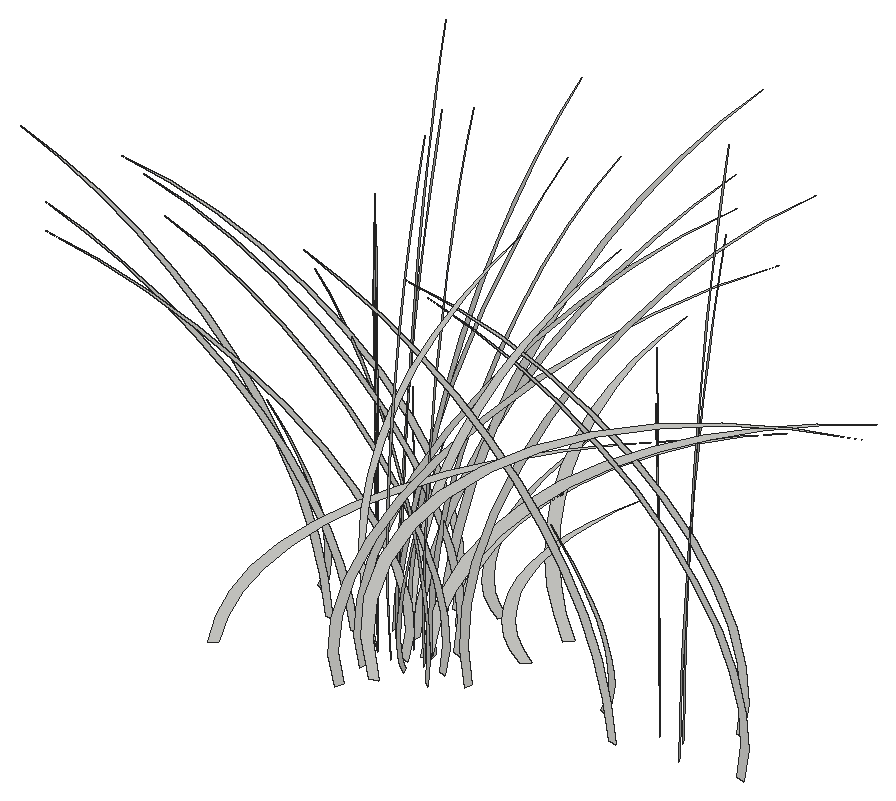
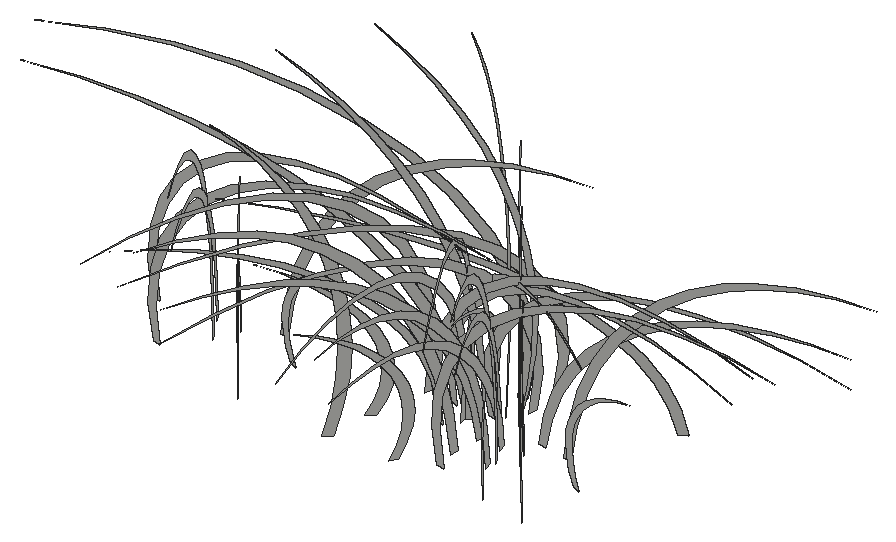
# SketchUp Ruby script. Lengths in inches.
U = 1.inch
M = Sketchup.active_model
def pt(a) = Geom::Point3d.new(a.map { |v| v * U })
def face(e, loops, mat)
  f = e.add_face(loops[0].map { |a| pt(a) })
  loops[1..].each { |l| e.add_face(l.map { |a| pt(a) }).erase! }
  f.material = f.back_material = mat if mat
  f
end
# faces: each face lists its corners as indices into pts; further lists are holes
def faces(e, pts, list, mat = nil) = list.each { |f| face(e, (f[0].is_a?(Array) ? f : [f]).map { |l| l.map { |i| pts[i] } }, mat) }
# xy, xz, yz: faces in a plane at the given z, y or x. An outline is a flat list of corners, or four numbers for a rectangle; further outlines are holes
def ring(l) = l.size == 4 ? [[l[0], l[1]], [l[2], l[1]], [l[2], l[3]], [l[0], l[3]]] : l.each_slice(2).to_a
def flat(e, list, mat, &to3) = list.each { |f| face(e, (f[0].is_a?(Array) ? f : [f]).map { |l| ring(l).map { |u, v| to3.(u, v) } }, mat) }
def xy(e, z, list, mat = nil) = flat(e, list, mat) { |x, y| [x, y, z] }
def xz(e, y, list, mat = nil) = flat(e, list, mat) { |x, z| [x, y, z] }
def yz(e, x, list, mat = nil) = flat(e, list, mat) { |y, z| [x, y, z] }
def lines(e, pts, list) = list.each { |a, b| e.add_line(pt(pts[a]), pt(pts[b])) }
# prism: a flat outline (further loops are holes) pulled along v
def prism(e, loops, v, mat = nil)
  f = face(e, loops, mat); d = Geom::Vector3d.new(v.map { |x| x * U })
  f.pushpull(f.normal.samedirection?(d) ? d.length : -d.length)
end
def box(e, o, s, mat = nil) = prism(e, [[o, [o[0] + s[0], o[1], o[2]], [o[0] + s[0], o[1] + s[1], o[2]], [o[0], o[1] + s[1], o[2]]]], [0, 0, s[2]], mat)
def at(x, y, z, deg = 0) = Geom::Transformation.translation(pt([x, y, z])) * Geom::Transformation.rotation(ORIGIN, Z_AXIS, deg.degrees)
def axes(o, x, y, z) = Geom::Transformation.new([*x, 0, *y, 0, *z, 0, *pt(o).to_a, 1])
def part(name) = M.definitions.add(name)
# library, detail: a bought-in or finely detailed component or shape, given as its bounding box
def library(name, o, s) = part(name).tap { |d| box(d.entities, o, s) }
def detail(e, o, s) = box(e.add_group.entities, o, s)
def put(e, d, t, mat = nil) = e.add_instance(d, t).tap { |i| i.material = mat if mat }
def group(e, t, mat = nil) = e.add_group.tap { |g| g.transformation = t; g.material = mat if mat }.entities
root = M.entities
g1 = group(root,at(381.84,271.38,0))
p = [[-20.46,3.64,18.05],[-23.54,4.19,18.53],[-20.55,3.66,17.95],[-17.67,3.15,17.15],[-14.91,2.66,16.14],[-12.33,2.2,14.93],
  [-9.93,1.77,13.53],[-7.76,1.38,11.96],[-5.84,1.04,10.23],[-4.18,0.74,8.37],[-2.8,0.5,6.39],[-1.73,0.31,4.32],
  [-0.97,0.17,2.18],[-0.53,0.09,0],[0,0,0],[-0.36,0.0625,2.23],[-1.07,0.19,4.43],[-2.125,0.38,6.55],
  [-3.51,0.625,8.57],[-5.2,0.93,10.47],[-7.1875,1.28,12.22],[-9.43,1.68,13.8],[-11.92,2.125,15.1875],[-14.61,2.6,16.37],
  [-17.46,3.11,17.33]]
faces(g1,p,[[0,1,2,3,4,5,6,7,8,9,10,11,12,13,14,15,16,17,18,19,20,21,22,23,24]])
g2 = group(root,at(359.18,266.76,0.02))
p = [[17.17,11.7,12.375],[19.76,13.47,12.7],[17.25,11.76,12.31],[14.83,10.11,11.76],[12.52,8.53,11.07],[10.35,7.05,10.23],
  [8.34,5.68,9.27],[6.52,4.44,8.2],[4.9,3.34,7.01],[3.51,2.39,5.74],[2.35,1.6,4.38],[1.45,0.99,2.96],
  [0.82,0.56,1.5],[0.45,0.3,0],[0,0,0],[0.3,0.21,1.53],[0.9,0.61,3.03],[1.78,1.22,4.49],
  [2.95,2.01,5.875],[4.37,2.98,7.18],[6.03,4.11,8.375],[7.92,5.4,9.46],[10,6.82,10.41],[12.26,8.36,11.22],
  [14.66,9.99,11.88]]
faces(g2,p,[[0,1,2,3,4,5,6,7,8,9,10,11,12,13,14,15,16,17,18,19,20,21,22,23,24]])
g3 = group(root,at(365.85,270.62,0.02))
p = [[0.67,0.67,0],[0.3,0.3,2.04],[0.08,0.08,4.1],[0,0,6.17],[0.07,0.07,8.23],[0.3,0.3,10.29],
  [0.66,0.66,12.33],[1.18,1.18,14.34],[1.84,1.84,16.32],[2.64,2.64,18.26],[3.58,3.58,20.14],[4.65,4.65,21.96],
  [5.84,5.84,23.71],[4.72,4.72,21.93],[3.71,3.71,20.09],[2.82,2.82,18.2],[2.05,2.05,16.26],[1.42,1.42,14.29],
  [0.91,0.91,12.29],[0.54,0.54,10.26],[0.3,0.3,8.21],[0.1875,0.1875,6.15],[0.22,0.22,4.09],[0.375,0.375,2.04]]
faces(g3,p,[[0,1,2,3,4,5,6,7,8,9,10,11,12,13,14,15,16,17,18,19,20,21,22,23]])
g4 = group(root,at(369.38,269.29,0.02))
p = [[-3.85,8.68,9.0625],[-3.11,7.03,8.49],[-2.45,5.54,7.85],[-1.87,4.22,7.18],[-1.37,3.08,6.45],[-0.95,2.15,5.7],
  [-0.625,1.41,4.91],[-0.39,0.89,4.1],[-0.26,0.58,3.28],[-0.22,0.49,2.45],[-0.28,0.625,1.625],[-0.43,0.97,0.8],
  [-0.68,1.54,0],[-0.52,1.16,0],[-0.23,0.52,0.8],[-0.05,0.11,1.61],[0.02,-0.06,2.45],[-0.01,0.02,3.28],
  [-0.15,0.33,4.11],[-0.39,0.89,4.93],[-0.74,1.67,5.72],[-1.1875,2.68,6.49],[-1.73,3.9,7.21],[-2.35,5.3125,7.88],
  [-3.0625,6.91,8.5]]
faces(g4,p,[[0,1,2,3,4,5,6,7,8,9,10,11,12,13,14,15,16,17,18,19,20,21,22,23,24]])
g5 = group(root,at(367.54,268.67,0.02))
p = [[0.85,0.36,0],[0.38,0.16,0],[0,0,2.37],[0.15,0.0625,4.75],[0.84,0.35,7.08],[2.03,0.85,9.32],
  [3.71,1.54,11.39],[5.83,2.42,13.25],[8.33,3.47,14.85],[11.16,4.65,16.15],[14.25,5.93,17.13],[17.52,7.29,17.75],
  [20.89,8.69,18.01],[24.27,10.1,17.89],[20.95,8.72,17.91],[17.67,7.35,17.58],[14.49,6.03,16.9],[11.5,4.79,15.89],
  [8.76,3.65,14.58],[6.33,2.63,12.99],[4.27,1.78,11.15],[2.63,1.1,9.125],[1.45,0.6,6.94],[0.75,0.3125,4.66],
  [0.55,0.23,2.33]]
faces(g5,p,[[0,1,2,3,4,5,6,7,8,9,10,11,12,13,14,15,16,17,18,19,20,21,22,23,24]])
g6 = group(root,at(367.12,270.56,0.02))
p = [[-0.6,0.73,0],[-0.27,0.33,1.77],[-0.07,0.08,3.57],[0,0,5.36],[-0.07,0.08,7.16],[-0.27,0.32,8.95],
  [-0.6,0.73,10.73],[-1.06,1.29,12.48],[-1.65,2.01,14.2],[-2.37,2.88,15.88],[-3.21,3.91,17.52],[-4.17,5.08,19.1],
  [-5.25,6.39,20.625],[-4.23,5.15,19.08],[-3.33,4.05,17.48],[-2.53,3.08,15.83],[-1.84,2.25,14.15],[-1.27,1.55,12.43],
  [-0.82,1,10.6875],[-0.48,0.59,8.92],[-0.27,0.32,7.14],[-0.17,0.21,5.35],[-0.19,0.24,3.5625],[-0.34,0.41,1.78]]
faces(g6,p,[[0,1,2,3,4,5,6,7,8,9,10,11,12,13,14,15,16,17,18,19,20,21,22,23]])
g7 = group(root,at(368.81,271.35,0.02))
p = [[-0.98,0.17,0],[-0.43,0.08,0],[0,0,1.75],[-0.18,0.03,3.51],[-0.96,0.17,5.24],[-2.32,0.41,6.89],
  [-4.24,0.76,8.42],[-6.67,1.1875,9.8],[-9.54,1.7,10.98],[-12.78,2.28,11.95],[-16.32,2.91,12.67],[-20.06,3.57,13.13],
  [-23.91,4.26,13.32],[-27.78,4.95,13.23],[-23.98,4.27,13.25],[-20.22,3.6,13],[-16.59,2.96,12.5],[-13.16,2.34,11.75],
  [-10.02,1.79,10.78],[-7.25,1.29,9.6],[-4.89,0.87,8.25],[-3.02,0.54,6.75],[-1.66,0.3,5.13],[-0.86,0.15,3.44],
  [-0.63,0.11,1.72]]
faces(g7,p,[[0,1,2,3,4,5,6,7,8,9,10,11,12,13,14,15,16,17,18,19,20,21,22,23,24]])
g8 = group(root,at(368.81,271.35,0.02))
p = [[-0.98,0.17,0],[-0.43,0.08,0],[0,0,1.75],[-0.18,0.03,3.51],[-0.96,0.17,5.24],[-2.32,0.41,6.89],
  [-4.24,0.76,8.42],[-6.67,1.1875,9.8],[-9.54,1.7,10.98],[-12.78,2.28,11.95],[-16.32,2.91,12.67],[-20.06,3.57,13.13],
  [-23.91,4.26,13.32],[-27.78,4.95,13.23],[-23.98,4.27,13.25],[-20.22,3.6,13],[-16.59,2.96,12.5],[-13.16,2.34,11.75],
  [-10.02,1.79,10.78],[-7.25,1.29,9.6],[-4.89,0.87,8.25],[-3.02,0.54,6.75],[-1.66,0.3,5.13],[-0.86,0.15,3.44],
  [-0.63,0.11,1.72]]
faces(g8,p,[[0,1,2,3,4,5,6,7,8,9,10,11,12,13,14,15,16,17,18,19,20,21,22,23,24]])
g9 = group(root,at(367.92,270.26,0.02))
p = [[-0.4,0.86,0],[-0.18,0.38,2.26],[-0.05,0.1,4.55],[0,0,6.84],[-0.04,0.09,9.14],[-0.18,0.38,11.42],
  [-0.4,0.85,13.6875],[-0.71,1.51,15.92],[-1.1,2.36,18.12],[-1.58,3.38,20.26],[-2.14,4.58,22.35],[-2.79,5.95,24.37],
  [-3.51,7.48,26.3125],[-2.83,6.04,24.34],[-2.22,4.75,22.3],[-1.69,3.61,20.2],[-1.23,2.63,18.05],[-0.85,1.82,15.86],
  [-0.55,1.17,13.64],[-0.32,0.6875,11.38],[-0.18,0.38,9.11],[-0.11,0.24,6.83],[-0.13,0.28,4.54],[-0.23,0.48,2.27]]
faces(g9,p,[[0,1,2,3,4,5,6,7,8,9,10,11,12,13,14,15,16,17,18,19,20,21,22,23]])
g10 = group(root,at(364.57,272.11,0.02))
p = [[-20.46,3.64,14.56],[-23.54,4.19,14.94],[-20.55,3.66,14.48],[-17.67,3.15,13.83],[-14.91,2.66,13.02],[-12.33,2.2,12.04],
  [-9.93,1.77,10.91],[-7.76,1.38,9.64],[-5.84,1.04,8.25],[-4.18,0.74,6.75],[-2.8,0.5,5.15],[-1.73,0.31,3.49],
  [-0.97,0.17,1.76],[-0.53,0.09,0],[0,0,0],[-0.36,0.0625,1.8],[-1.07,0.19,3.57],[-2.125,0.38,5.28],
  [-3.51,0.625,6.91],[-5.2,0.93,8.44],[-7.1875,1.28,9.85],[-9.43,1.68,11.13],[-11.92,2.125,12.25],[-14.61,2.6,13.2],
  [-17.46,3.11,13.97]]
faces(g10,p,[[0,1,2,3,4,5,6,7,8,9,10,11,12,13,14,15,16,17,18,19,20,21,22,23,24]])
g11 = group(root,at(362.67,272.45,0.02))
p = [[-20.46,3.64,18.05],[-23.54,4.19,18.53],[-20.55,3.66,17.95],[-17.67,3.15,17.15],[-14.91,2.66,16.14],[-12.33,2.2,14.93],
  [-9.93,1.77,13.53],[-7.76,1.38,11.96],[-5.84,1.04,10.23],[-4.18,0.74,8.37],[-2.8,0.5,6.39],[-1.73,0.31,4.32],
  [-0.97,0.17,2.18],[-0.53,0.09,0],[0,0,0],[-0.36,0.0625,2.23],[-1.07,0.19,4.43],[-2.125,0.38,6.55],
  [-3.51,0.625,8.57],[-5.2,0.93,10.47],[-7.1875,1.28,12.22],[-9.43,1.68,13.8],[-11.92,2.125,15.1875],[-14.61,2.6,16.37],
  [-17.46,3.11,17.33]]
faces(g11,p,[[0,1,2,3,4,5,6,7,8,9,10,11,12,13,14,15,16,17,18,19,20,21,22,23,24]])
g12 = group(root,at(380.4,273.07,0))
p = [[-6.53,2.99,7.88],[-5.33,2.44,7.38],[-4.26,1.95,6.83],[-3.3,1.51,6.24],[-2.48,1.14,5.62],[-1.81,0.83,4.96],
  [-1.28,0.58,4.27],[-0.9,0.41,3.57],[-0.68,0.31,2.86],[-0.61,0.28,2.13],[-0.71,0.32,1.41],[-0.96,0.4375,0.7],
  [-1.37,0.625,0],[-0.84,0.38,0],[-0.39,0.18,0.71],[-0.11,0.05,1.43],[0,0,2.17],[-0.07,0.03,2.9],
  [-0.32,0.15,3.63],[-0.74,0.34,4.34],[-1.33,0.61,5.03],[-2.08,0.95,5.69],[-2.99,1.37,6.3125],[-4.04,1.85,6.89],
  [-5.22,2.39,7.41]]
faces(g12,p,[[0,1,2,3,4,5,6,7,8,9,10,11,12,13,14,15,16,17,18,19,20,21,22,23,24]])
g13 = group(root,at(361.23,274.14,0.02))
p = [[-6.53,2.99,7.88],[-5.33,2.44,7.38],[-4.26,1.95,6.83],[-3.3,1.51,6.24],[-2.48,1.14,5.62],[-1.81,0.83,4.96],
  [-1.28,0.58,4.27],[-0.9,0.41,3.57],[-0.68,0.31,2.86],[-0.61,0.28,2.13],[-0.71,0.32,1.41],[-0.96,0.4375,0.7],
  [-1.37,0.625,0],[-0.84,0.38,0],[-0.39,0.18,0.71],[-0.11,0.05,1.43],[0,0,2.17],[-0.07,0.03,2.9],
  [-0.32,0.15,3.63],[-0.74,0.34,4.34],[-1.33,0.61,5.03],[-2.08,0.95,5.69],[-2.99,1.37,6.3125],[-4.04,1.85,6.89],
  [-5.22,2.39,7.41]]
faces(g13,p,[[0,1,2,3,4,5,6,7,8,9,10,11,12,13,14,15,16,17,18,19,20,21,22,23,24]])
g14 = group(root,at(370.99,269.92,0.02))
p = [[-0.62,0.44,0],[-0.27,0.2,0],[0,0,1.68],[-0.11,0.08,3.37],[-0.6,0.43,5.03],[-1.46,1.05,6.61],
  [-2.67,1.92,8.08],[-4.2,3.02,9.4],[-6.01,4.32,10.54],[-8.05,5.79,11.47],[-10.28,7.39,12.16],[-12.64,9.08,12.61],
  [-15.07,10.83,12.79],[-17.5,12.58,12.7],[-15.11,10.86,12.72],[-12.74,9.16,12.48],[-10.45,7.51,12],[-8.29,5.96,11.29],
  [-6.32,4.54,10.35],[-4.57,3.28,9.22],[-3.08,2.21,7.92],[-1.9,1.37,6.48],[-1.05,0.75,4.93],[-0.54,0.39,3.31],
  [-0.4,0.29,1.65]]
faces(g14,p,[[0,1,2,3,4,5,6,7,8,9,10,11,12,13,14,15,16,17,18,19,20,21,22,23,24]])
g15 = group(root,at(367.73,272.5,0.02))
p = [[7.51,7.51,22.54],[6.3125,6.3125,20.88],[5.21,5.21,19.16],[4.21,4.21,17.39],[3.32,3.32,15.57],[2.52,2.52,13.71],
  [1.84,1.84,11.82],[1.27,1.27,9.89],[0.81,0.81,7.94],[0.46,0.46,5.97],[0.22,0.22,3.99],[0.1,0.1,2],
  [0.1,0.1,0],[0,0,2.01],[0.04,0.04,4.01],[0.21,0.21,6.01],[0.51,0.51,8],[0.95,0.95,9.97],
  [1.51,1.51,11.91],[2.21,2.21,13.81],[3.03,3.03,15.67],[3.98,3.98,17.48],[5.04,5.04,19.23],[6.22,6.22,20.92]]
faces(g15,p,[[0,1,2,3,4,5,6,7,8,9,10,11,12,13,14,15,16,17,18,19,20,21,22,23]])
g16 = group(root,at(389.66,272.32,0))
p = [[-0.95,0.28,0],[-0.42,0.125,0],[0,0,2.01],[-0.17,0.05,4.04],[-0.93,0.27,6.02],[-2.27,0.66,7.92],
  [-4.14,1.21,9.68],[-6.5,1.9,11.26],[-9.3,2.72,12.62],[-12.46,3.64,13.73],[-15.91,4.65,14.5625],[-19.55,5.72,15.09],
  [-23.3125,6.82,15.31],[-27.08,7.92,15.2],[-23.38,6.84,15.22],[-19.72,5.77,14.94],[-16.17,4.73,14.37],[-12.83,3.75,13.51],
  [-9.77,2.86,12.39],[-7.0625,2.07,11.04],[-4.77,1.39,9.48],[-2.94,0.86,7.75],[-1.62,0.47,5.9],[-0.84,0.25,3.96],
  [-0.61,0.18,1.98]]
faces(g16,p,[[0,1,2,3,4,5,6,7,8,9,10,11,12,13,14,15,16,17,18,19,20,21,22,23,24]])
g17 = group(root,at(371.15,271.3125,0.02))
p = [[-0.93,0.35,0],[-0.41,0.16,0],[0,0,1.75],[-0.17,0.0625,3.51],[-0.91,0.34,5.24],[-2.21,0.83,6.89],
  [-4.03,1.52,8.42],[-6.34,2.39,9.8],[-9.0625,3.42,10.98],[-12.14,4.59,11.95],[-15.5,5.86,12.67],[-19.06,7.2,13.13],
  [-22.72,8.58,13.32],[-26.4,9.97,13.23],[-22.79,8.61,13.25],[-19.22,7.26,13],[-15.76,5.96,12.5],[-12.51,4.73,11.75],
  [-9.53,3.6,10.78],[-6.89,2.6,9.6],[-4.65,1.76,8.25],[-2.87,1.08,6.75],[-1.58,0.6,5.13],[-0.82,0.31,3.44],
  [-0.6,0.23,1.72]]
faces(g17,p,[[0,1,2,3,4,5,6,7,8,9,10,11,12,13,14,15,16,17,18,19,20,21,22,23,24]])
g18 = group(root,at(365.43,272.61,0.02))
p = [[-6.74,8.21,19.61],[-5.67,6.9,18.16],[-4.68,5.7,16.67],[-3.78,4.6,15.125],[-2.98,3.62,13.55],[-2.27,2.76,11.93],
  [-1.65,2.01,10.28],[-1.14,1.39,8.61],[-0.72,0.88,6.91],[-0.41,0.5,5.2],[-0.2,0.24,3.47],[-0.09,0.11,1.74],
  [-0.09,0.11,0],[0,0,1.74],[-0.03,0.04,3.49],[-0.1875,0.23,5.23],[-0.46,0.56,6.96],[-0.85,1.04,8.67],
  [-1.36,1.66,10.36],[-1.98,2.42,12.01],[-2.72,3.3125,13.63],[-3.57,4.35,15.21],[-4.52,5.51,16.73],[-5.58,6.8,18.2]]
faces(g18,p,[[0,1,2,3,4,5,6,7,8,9,10,11,12,13,14,15,16,17,18,19,20,21,22,23]])
g19 = group(root,at(365.43,272.61,0.02))
p = [[-6.74,8.21,19.61],[-5.67,6.9,18.16],[-4.68,5.7,16.67],[-3.78,4.6,15.125],[-2.98,3.62,13.55],[-2.27,2.76,11.93],
  [-1.65,2.01,10.28],[-1.14,1.39,8.61],[-0.72,0.88,6.91],[-0.41,0.5,5.2],[-0.2,0.24,3.47],[-0.09,0.11,1.74],
  [-0.09,0.11,0],[0,0,1.74],[-0.03,0.04,3.49],[-0.1875,0.23,5.23],[-0.46,0.56,6.96],[-0.85,1.04,8.67],
  [-1.36,1.66,10.36],[-1.98,2.42,12.01],[-2.72,3.3125,13.63],[-3.57,4.35,15.21],[-4.52,5.51,16.73],[-5.58,6.8,18.2]]
faces(g19,p,[[0,1,2,3,4,5,6,7,8,9,10,11,12,13,14,15,16,17,18,19,20,21,22,23]])
g20 = group(root,at(372.19,274.23,0.02))
p = [[5.08,5.08,9.0625],[4.15,4.15,8.49],[3.31,3.31,7.85],[2.57,2.57,7.18],[1.93,1.93,6.45],[1.41,1.41,5.7],
  [0.99,0.99,4.91],[0.7,0.7,4.1],[0.53,0.53,3.28],[0.48,0.48,2.45],[0.55,0.55,1.625],[0.75,0.75,0.8],
  [1.0625,1.0625,0],[0.65,0.65,0],[0.3,0.3,0.81],[0.08,0.08,1.65],[0,0,2.49],[0.06,0.06,3.34],
  [0.25,0.25,4.17],[0.58,0.58,4.99],[1.04,1.04,5.79],[1.62,1.62,6.54],[2.33,2.33,7.26],[3.14,3.14,7.92],
  [4.0625,4.0625,8.52]]
faces(g20,p,[[0,1,2,3,4,5,6,7,8,9,10,11,12,13,14,15,16,17,18,19,20,21,22,23,24]])
g21 = group(root,at(368.57,272.24,0.02))
p = [[19.18,7.98,16.73],[22.08,9.1875,17.17],[19.27,8.02,16.64],[16.57,6.9,15.9],[13.98,5.82,14.96],[11.56,4.8125,13.84],
  [9.32,3.88,12.54],[7.28,3.03,11.08],[5.47,2.28,9.48],[3.92,1.63,7.76],[2.63,1.09,5.92],[1.625,0.68,4.01],
  [0.91,0.38,2.02],[0.5,0.21,0],[0,0,0],[0.34,0.14,2.07],[1.01,0.42,4.1],[1.99,0.83,6.07],
  [3.29,1.37,7.94],[4.88,2.03,9.7],[6.74,2.81,11.33],[8.85,3.68,12.79],[11.18,4.65,14.08],[13.7,5.7,15.17],
  [16.375,6.82,16.0625]]
faces(g21,p,[[0,1,2,3,4,5,6,7,8,9,10,11,12,13,14,15,16,17,18,19,20,21,22,23,24]])
g22 = group(root,at(370.49,273.39,0.02))
p = [[-0.95,0.28,0],[-0.42,0.125,0],[0,0,2.01],[-0.17,0.05,4.04],[-0.93,0.27,6.02],[-2.27,0.66,7.92],
  [-4.14,1.21,9.68],[-6.5,1.9,11.26],[-9.3,2.72,12.62],[-12.46,3.64,13.73],[-15.91,4.65,14.5625],[-19.55,5.72,15.09],
  [-23.3125,6.82,15.31],[-27.08,7.92,15.2],[-23.38,6.84,15.22],[-19.72,5.77,14.94],[-16.17,4.73,14.37],[-12.83,3.75,13.51],
  [-9.77,2.86,12.39],[-7.0625,2.07,11.04],[-4.77,1.39,9.48],[-2.94,0.86,7.75],[-1.62,0.47,5.9],[-0.84,0.25,3.96],
  [-0.61,0.18,1.98]]
faces(g22,p,[[0,1,2,3,4,5,6,7,8,9,10,11,12,13,14,15,16,17,18,19,20,21,22,23,24]])
g23 = group(root,at(386.81,275.89,0))
p = [[-0.91,0.16,0],[-0.4,0.07,0],[0,0,2.0625],[-0.16,0.03,4.13],[-0.89,0.16,6.16],[-2.17,0.39,8.1],
  [-3.95,0.7,9.91],[-6.21,1.11,11.52],[-8.88,1.58,12.92],[-11.91,2.12,14.05],[-15.2,2.71,14.9],[-18.68,3.33,15.45],
  [-22.27,3.97,15.67],[-25.88,4.61,15.5625],[-22.34,3.98,15.58],[-18.84,3.36,15.29],[-15.45,2.75,14.71],[-12.26,2.18,13.83],
  [-9.34,1.66,12.68],[-6.75,1.2,11.3],[-4.56,0.8125,9.7],[-2.81,0.5,7.9375],[-1.55,0.28,6.04],[-0.8,0.14,4.05],
  [-0.59,0.1,2.02]]
faces(g23,p,[[0,1,2,3,4,5,6,7,8,9,10,11,12,13,14,15,16,17,18,19,20,21,22,23,24]])
g24 = group(root,at(386.81,275.89,0))
p = [[-0.91,0.16,0],[-0.4,0.07,0],[0,0,2.0625],[-0.16,0.03,4.13],[-0.89,0.16,6.16],[-2.17,0.39,8.1],
  [-3.95,0.7,9.91],[-6.21,1.11,11.52],[-8.88,1.58,12.92],[-11.91,2.12,14.05],[-15.2,2.71,14.9],[-18.68,3.33,15.45],
  [-22.27,3.97,15.67],[-25.88,4.61,15.5625],[-22.34,3.98,15.58],[-18.84,3.36,15.29],[-15.45,2.75,14.71],[-12.26,2.18,13.83],
  [-9.34,1.66,12.68],[-6.75,1.2,11.3],[-4.56,0.8125,9.7],[-2.81,0.5,7.9375],[-1.55,0.28,6.04],[-0.8,0.14,4.05],
  [-0.59,0.1,2.02]]
faces(g24,p,[[0,1,2,3,4,5,6,7,8,9,10,11,12,13,14,15,16,17,18,19,20,21,22,23,24]])
g25 = group(root,at(367.64,276.95,0.02))
p = [[-0.91,0.16,0],[-0.4,0.07,0],[0,0,2.0625],[-0.16,0.03,4.13],[-0.89,0.16,6.16],[-2.17,0.39,8.1],
  [-3.95,0.7,9.91],[-6.21,1.11,11.52],[-8.88,1.58,12.92],[-11.91,2.12,14.05],[-15.2,2.71,14.9],[-18.68,3.33,15.45],
  [-22.27,3.97,15.67],[-25.88,4.61,15.5625],[-22.34,3.98,15.58],[-18.84,3.36,15.29],[-15.45,2.75,14.71],[-12.26,2.18,13.83],
  [-9.34,1.66,12.68],[-6.75,1.2,11.3],[-4.56,0.8125,9.7],[-2.81,0.5,7.9375],[-1.55,0.28,6.04],[-0.8,0.14,4.05],
  [-0.59,0.1,2.02]]
faces(g25,p,[[0,1,2,3,4,5,6,7,8,9,10,11,12,13,14,15,16,17,18,19,20,21,22,23,24]])
g26 = group(root,at(367.64,276.95,0.02))
p = [[-0.91,0.16,0],[-0.4,0.07,0],[0,0,2.0625],[-0.16,0.03,4.13],[-0.89,0.16,6.16],[-2.17,0.39,8.1],
  [-3.95,0.7,9.91],[-6.21,1.11,11.52],[-8.88,1.58,12.92],[-11.91,2.12,14.05],[-15.2,2.71,14.9],[-18.68,3.33,15.45],
  [-22.27,3.97,15.67],[-25.88,4.61,15.5625],[-22.34,3.98,15.58],[-18.84,3.36,15.29],[-15.45,2.75,14.71],[-12.26,2.18,13.83],
  [-9.34,1.66,12.68],[-6.75,1.2,11.3],[-4.56,0.8125,9.7],[-2.81,0.5,7.9375],[-1.55,0.28,6.04],[-0.8,0.14,4.05],
  [-0.59,0.1,2.02]]
faces(g26,p,[[0,1,2,3,4,5,6,7,8,9,10,11,12,13,14,15,16,17,18,19,20,21,22,23,24]])
g27 = group(root,at(380.29,276.79,0))
p = [[-4.56,5.55,16.02],[-3.72,4.53,15.01],[-2.97,3.62,13.89],[-2.31,2.81,12.69],[-1.73,2.11,11.42],[-1.26,1.54,10.08],
  [-0.89,1.09,8.6875],[-0.63,0.76,7.26],[-0.47,0.58,5.8],[-0.43,0.52,4.34],[-0.49,0.6,2.87],[-0.67,0.81,1.42],
  [-0.95,1.16,0],[-0.59,0.71,0],[-0.27,0.33,1.44],[-0.07,0.09,2.92],[0,0,4.41],[-0.05,0.0625,5.9],
  [-0.22,0.27,7.38],[-0.52,0.63,8.83],[-0.93,1.13,10.23],[-1.45,1.77,11.57],[-2.09,2.54,12.83],[-2.82,3.43,14.01],
  [-3.65,4.44,15.07]]
faces(g27,p,[[0,1,2,3,4,5,6,7,8,9,10,11,12,13,14,15,16,17,18,19,20,21,22,23,24]])
g28 = group(root,at(380.29,276.79,0))
p = [[-4.56,5.55,16.02],[-3.72,4.53,15.01],[-2.97,3.62,13.89],[-2.31,2.81,12.69],[-1.73,2.11,11.42],[-1.26,1.54,10.08],
  [-0.89,1.09,8.6875],[-0.63,0.76,7.26],[-0.47,0.58,5.8],[-0.43,0.52,4.34],[-0.49,0.6,2.87],[-0.67,0.81,1.42],
  [-0.95,1.16,0],[-0.59,0.71,0],[-0.27,0.33,1.44],[-0.07,0.09,2.92],[0,0,4.41],[-0.05,0.0625,5.9],
  [-0.22,0.27,7.38],[-0.52,0.63,8.83],[-0.93,1.13,10.23],[-1.45,1.77,11.57],[-2.09,2.54,12.83],[-2.82,3.43,14.01],
  [-3.65,4.44,15.07]]
faces(g28,p,[[0,1,2,3,4,5,6,7,8,9,10,11,12,13,14,15,16,17,18,19,20,21,22,23,24]])
g29 = group(root,at(383.16,273.3,0))
p = [[-10.66,12.98,9.9],[-9.23,11.23,9.83],[-7.82,9.52,9.59],[-6.46,7.86,9.18],[-5.18,6.3,8.61],[-3.99,4.86,7.88],
  [-2.93,3.57,7.02],[-2.02,2.46,6.03],[-1.27,1.54,4.95],[-0.6875,0.84,3.78],[-0.29,0.36,2.55],[-0.1,0.12,1.28],
  [-0.09,0.12,0],[0,0,1.3],[-0.125,0.15,2.61],[-0.47,0.57,3.875],[-1.02,1.24,5.09],[-1.77,2.15,6.21],
  [-2.69,3.28,7.22],[-3.78,4.6,8.1],[-5,6.09,8.82],[-6.33,7.71,9.37],[-7.74,9.43,9.74],[-9.2,11.19,9.92]]
faces(g29,p,[[0,1,2,3,4,5,6,7,8,9,10,11,12,13,14,15,16,17,18,19,20,21,22,23]])
g30 = group(root,at(372.53,277.3,0.02))
p = [[5.08,5.08,18.42],[4.15,4.15,17.25],[3.31,3.31,15.97],[2.57,2.57,14.59],[1.93,1.93,13.12],[1.41,1.41,11.58],
  [0.99,0.99,9.98],[0.7,0.7,8.34],[0.53,0.53,6.67],[0.48,0.48,4.99],[0.55,0.55,3.3],[0.75,0.75,1.63],
  [1.0625,1.0625,0],[0.65,0.65,0],[0.3,0.3,1.66],[0.08,0.08,3.35],[0,0,5.07],[0.06,0.06,6.79],
  [0.25,0.25,8.49],[0.58,0.58,10.15],[1.04,1.04,11.76],[1.62,1.62,13.3],[2.33,2.33,14.75],[3.14,3.14,16.1],
  [4.0625,4.0625,17.33]]
faces(g30,p,[[0,1,2,3,4,5,6,7,8,9,10,11,12,13,14,15,16,17,18,19,20,21,22,23,24]])
g31 = group(root,at(364.15,277.22,0.02))
p = [[-4.56,5.55,7.88],[-3.72,4.53,7.38],[-2.97,3.62,6.83],[-2.31,2.81,6.24],[-1.73,2.11,5.62],[-1.26,1.54,4.96],
  [-0.89,1.09,4.27],[-0.63,0.76,3.57],[-0.47,0.58,2.86],[-0.43,0.52,2.13],[-0.49,0.6,1.41],[-0.67,0.81,0.7],
  [-0.95,1.16,0],[-0.59,0.71,0],[-0.27,0.33,0.71],[-0.07,0.09,1.43],[0,0,2.17],[-0.05,0.0625,2.9],
  [-0.22,0.27,3.63],[-0.52,0.63,4.34],[-0.93,1.13,5.03],[-1.45,1.77,5.69],[-2.09,2.54,6.3125],[-2.82,3.43,6.89],
  [-3.65,4.44,7.41]]
faces(g31,p,[[0,1,2,3,4,5,6,7,8,9,10,11,12,13,14,15,16,17,18,19,20,21,22,23,24]])
g32 = group(root,at(369.34,274.11,0.02))
p = [[11.88,11.88,11.375],[10.28,10.28,11.3],[8.71,8.71,11.03],[7.19,7.19,10.55],[5.77,5.77,9.89],[4.45,4.45,9.0625],
  [3.27,3.27,8.07],[2.25,2.25,6.9375],[1.41,1.41,5.69],[0.76,0.76,4.34],[0.33,0.33,2.93],[0.11,0.11,1.47],
  [0.11,0.11,0],[0,0,1.5],[0.14,0.14,3],[0.52,0.52,4.46],[1.13,1.13,5.85],[1.97,1.97,7.14],
  [3,3,8.3],[4.21,4.21,9.31],[5.58,5.58,10.14],[7.06,7.06,10.77],[8.625,8.625,11.19],[10.24,10.24,11.4]]
faces(g32,p,[[0,1,2,3,4,5,6,7,8,9,10,11,12,13,14,15,16,17,18,19,20,21,22,23]])
g33 = group(root,at(368.84,276.84,0.02))
p = [[2.34,6.79,9.0625],[1.91,5.55,8.49],[1.52,4.43,7.85],[1.18,3.44,7.18],[0.89,2.58,6.45],[0.65,1.88,5.7],
  [0.46,1.33,4.91],[0.32,0.93,4.1],[0.24,0.7,3.28],[0.22,0.64,2.45],[0.25,0.74,1.625],[0.34,1,0.8],
  [0.49,1.42,0],[0.3,0.875,0],[0.14,0.4,0.81],[0.04,0.11,1.65],[0,0,2.49],[0.03,0.07,3.34],
  [0.11,0.33,4.17],[0.27,0.77,4.99],[0.48,1.38,5.79],[0.75,2.17,6.54],[1.07,3.11,7.26],[1.45,4.2,7.92],
  [1.87,5.43,8.52]]
faces(g33,p,[[0,1,2,3,4,5,6,7,8,9,10,11,12,13,14,15,16,17,18,19,20,21,22,23,24]])
g34 = group(root,at(366.99,266.68,0.02))
p = [[0.26,0.96,0],[0.11,0.43,0],[0,0,2.01],[0.05,0.17,4.04],[0.25,0.9375,6.02],[0.62,2.28,7.92],
  [1.125,4.16,9.68],[1.76,6.54,11.26],[2.52,9.35,12.62],[3.38,12.53,13.73],[4.32,16,14.5625],[5.31,19.67,15.09],
  [6.33,23.45,15.31],[7.35,27.24,15.2],[6.35,23.52,15.22],[5.35,19.83,14.94],[4.39,16.27,14.37],[3.48,12.91,13.51],
  [2.65,9.83,12.39],[1.92,7.11,11.04],[1.29,4.8,9.48],[0.8,2.96,7.75],[0.44,1.63,5.9],[0.23,0.84,3.96],
  [0.17,0.62,1.98]]
faces(g34,p,[[0,1,2,3,4,5,6,7,8,9,10,11,12,13,14,15,16,17,18,19,20,21,22,23,24]])
g35 = group(root,at(361.12,277.86,0.02))
p = [[-4.56,5.55,16.02],[-3.72,4.53,15.01],[-2.97,3.62,13.89],[-2.31,2.81,12.69],[-1.73,2.11,11.42],[-1.26,1.54,10.08],
  [-0.89,1.09,8.6875],[-0.63,0.76,7.26],[-0.47,0.58,5.8],[-0.43,0.52,4.34],[-0.49,0.6,2.87],[-0.67,0.81,1.42],
  [-0.95,1.16,0],[-0.59,0.71,0],[-0.27,0.33,1.44],[-0.07,0.09,2.92],[0,0,4.41],[-0.05,0.0625,5.9],
  [-0.22,0.27,7.38],[-0.52,0.63,8.83],[-0.93,1.13,10.23],[-1.45,1.77,11.57],[-2.09,2.54,12.83],[-2.82,3.43,14.01],
  [-3.65,4.44,15.07]]
faces(g35,p,[[0,1,2,3,4,5,6,7,8,9,10,11,12,13,14,15,16,17,18,19,20,21,22,23,24]])
g36 = group(root,at(361.12,277.86,0.02))
p = [[-4.56,5.55,16.02],[-3.72,4.53,15.01],[-2.97,3.62,13.89],[-2.31,2.81,12.69],[-1.73,2.11,11.42],[-1.26,1.54,10.08],
  [-0.89,1.09,8.6875],[-0.63,0.76,7.26],[-0.47,0.58,5.8],[-0.43,0.52,4.34],[-0.49,0.6,2.87],[-0.67,0.81,1.42],
  [-0.95,1.16,0],[-0.59,0.71,0],[-0.27,0.33,1.44],[-0.07,0.09,2.92],[0,0,4.41],[-0.05,0.0625,5.9],
  [-0.22,0.27,7.38],[-0.52,0.63,8.83],[-0.93,1.13,10.23],[-1.45,1.77,11.57],[-2.09,2.54,12.83],[-2.82,3.43,14.01],
  [-3.65,4.44,15.07]]
faces(g36,p,[[0,1,2,3,4,5,6,7,8,9,10,11,12,13,14,15,16,17,18,19,20,21,22,23,24]])
g37 = group(root,at(363.99,274.37,0.02))
p = [[-10.66,12.98,9.9],[-9.23,11.23,9.83],[-7.82,9.52,9.59],[-6.46,7.86,9.18],[-5.18,6.3,8.61],[-3.99,4.86,7.88],
  [-2.93,3.57,7.02],[-2.02,2.46,6.03],[-1.27,1.54,4.95],[-0.6875,0.84,3.78],[-0.29,0.36,2.55],[-0.1,0.12,1.28],
  [-0.09,0.12,0],[0,0,1.3],[-0.125,0.15,2.61],[-0.47,0.57,3.875],[-1.02,1.24,5.09],[-1.77,2.15,6.21],
  [-2.69,3.28,7.22],[-3.78,4.6,8.1],[-5,6.09,8.82],[-6.33,7.71,9.37],[-7.74,9.43,9.74],[-9.2,11.19,9.92]]
faces(g37,p,[[0,1,2,3,4,5,6,7,8,9,10,11,12,13,14,15,16,17,18,19,20,21,22,23]])
g38 = group(root,at(385.46,271.95,0))
p = [[-11.32,17.43,16.73],[-13.02,20.05,17.17],[-11.37,17.51,16.64],[-9.77,15.05,15.9],[-8.25,12.7,14.96],[-6.82,10.5,13.84],
  [-5.5,8.46,12.54],[-4.29,6.61,11.08],[-3.23,4.97,9.48],[-2.3125,3.56,7.76],[-1.55,2.39,5.92],[-0.96,1.47,4.01],
  [-0.54,0.83,2.02],[-0.29,0.45,0],[0,0,0],[-0.2,0.31,2.07],[-0.59,0.91,4.1],[-1.18,1.8125,6.07],
  [-1.94,2.99,7.94],[-2.88,4.43,9.7],[-3.98,6.12,11.33],[-5.22,8.04,12.79],[-6.59,10.15,14.08],[-8.08,12.44,15.17],
  [-9.66,14.88,16.0625]]
faces(g38,p,[[0,1,2,3,4,5,6,7,8,9,10,11,12,13,14,15,16,17,18,19,20,21,22,23,24]])
g39 = group(root,at(369.51,271.2,0.02))
p = [[-0.5,0.78,0],[-0.22,0.34,0],[0,0,2.37],[-0.09,0.14,4.75],[-0.49,0.76,7.08],[-1.2,1.84,9.32],
  [-2.1875,3.37,11.39],[-3.4375,5.29,13.25],[-4.92,7.57,14.85],[-6.59,10.14,16.15],[-8.41,12.95,17.13],[-10.34,15.92,17.75],
  [-12.32,18.97,18.01],[-14.32,22.05,17.89],[-12.36,19.03,17.91],[-10.42,16.05,17.58],[-8.55,13.16,16.9],[-6.78,10.45,15.89],
  [-5.17,7.96,14.58],[-3.73,5.75,12.99],[-2.52,3.88,11.15],[-1.55,2.39,9.125],[-0.86,1.32,6.94],[-0.44,0.68,4.66],
  [-0.33,0.5,2.33]]
faces(g39,p,[[0,1,2,3,4,5,6,7,8,9,10,11,12,13,14,15,16,17,18,19,20,21,22,23,24]])
g40 = group(root,at(366.29,273.02,0.02))
p = [[-11.32,17.43,16.73],[-13.02,20.05,17.17],[-11.37,17.51,16.64],[-9.77,15.05,15.9],[-8.25,12.7,14.96],[-6.82,10.5,13.84],
  [-5.5,8.46,12.54],[-4.29,6.61,11.08],[-3.23,4.97,9.48],[-2.3125,3.56,7.76],[-1.55,2.39,5.92],[-0.96,1.47,4.01],
  [-0.54,0.83,2.02],[-0.29,0.45,0],[0,0,0],[-0.2,0.31,2.07],[-0.59,0.91,4.1],[-1.18,1.8125,6.07],
  [-1.94,2.99,7.94],[-2.88,4.43,9.7],[-3.98,6.12,11.33],[-5.22,8.04,12.79],[-6.59,10.15,14.08],[-8.08,12.44,15.17],
  [-9.66,14.88,16.0625]]
faces(g40,p,[[0,1,2,3,4,5,6,7,8,9,10,11,12,13,14,15,16,17,18,19,20,21,22,23,24]])
g41 = group(root,at(366.81,269.02,0.02))
p = [[0.08,0.99,0],[0.03,0.44,0],[0,0,2.01],[0.01,0.18,4.04],[0.08,0.97,6.02],[0.19,2.35,7.92],
  [0.34,4.3,9.68],[0.53,6.75,11.26],[0.76,9.66,12.62],[1.02,12.94,13.73],[1.3,16.52,14.5625],[1.6,20.31,15.09],
  [1.91,24.21,15.31],[2.21,28.13,15.2],[1.91,24.29,15.22],[1.61,20.48,14.94],[1.32,16.8,14.37],[1.05,13.33,13.51],
  [0.8,10.15,12.39],[0.58,7.34,11.04],[0.39,4.95,9.48],[0.24,3.05,7.75],[0.13,1.68,5.9],[0.07,0.87,3.96],
  [0.05,0.64,1.98]]
faces(g41,p,[[0,1,2,3,4,5,6,7,8,9,10,11,12,13,14,15,16,17,18,19,20,21,22,23,24]])
g42 = group(root,at(384.41,273.57,0))
p = [[-11.32,17.43,20.75],[-13.02,20.05,21.3],[-11.37,17.51,20.63],[-9.77,15.05,19.72],[-8.25,12.7,18.55],[-6.82,10.5,17.16],
  [-5.5,8.46,15.55],[-4.29,6.61,13.74],[-3.23,4.97,11.76],[-2.3125,3.56,9.62],[-1.55,2.39,7.35],[-0.96,1.47,4.97],
  [-0.54,0.83,2.51],[-0.29,0.45,0],[0,0,0],[-0.2,0.31,2.57],[-0.59,0.91,5.09],[-1.18,1.8125,7.53],
  [-1.94,2.99,9.85],[-2.88,4.43,12.03],[-3.98,6.12,14.04],[-5.22,8.04,15.86],[-6.59,10.15,17.46],[-8.08,12.44,18.82],
  [-9.66,14.88,19.92]]
faces(g42,p,[[0,1,2,3,4,5,6,7,8,9,10,11,12,13,14,15,16,17,18,19,20,21,22,23,24]])
g43 = group(root,at(372.27,270.73,0.02))
p = [[0.07,0.92,0],[0.03,0.41,0],[0,0,2.37],[0.01,0.17,4.75],[0.07,0.9,7.08],[0.17,2.19,9.32],
  [0.32,4,11.39],[0.5,6.29,13.25],[0.71,9,14.85],[0.95,12.06,16.15],[1.21,15.39,17.13],[1.49,18.92,17.75],
  [1.78,22.55,18.01],[2.0625,26.21,17.89],[1.78,22.625,17.91],[1.5,19.08,17.58],[1.23,15.65,16.9],[0.98,12.42,15.89],
  [0.74,9.46,14.58],[0.54,6.84,12.99],[0.36,4.61,11.15],[0.22,2.84,9.125],[0.125,1.57,6.94],[0.0625,0.8125,4.66],
  [0.05,0.59,2.33]]
faces(g43,p,[[0,1,2,3,4,5,6,7,8,9,10,11,12,13,14,15,16,17,18,19,20,21,22,23,24]])
g44 = group(root,at(369.23,272.05,0.02))
p = [[-0.27,0.88,0],[-0.12,0.39,0],[0,0,2.0625],[-0.05,0.16,4.13],[-0.26,0.87,6.16],[-0.64,2.1,8.1],
  [-1.17,3.84,9.91],[-1.84,6.03,11.52],[-2.64,8.63,12.92],[-3.54,11.5625,14.05],[-4.51,14.76,14.9],[-5.55,18.15,15.45],
  [-6.61,21.64,15.67],[-7.69,25.14,15.5625],[-6.63,21.7,15.58],[-5.59,18.3,15.29],[-4.59,15.01,14.71],[-3.64,11.91,13.83],
  [-2.77,9.07,12.68],[-2,6.56,11.3],[-1.35,4.43,9.7],[-0.83,2.73,7.9375],[-0.46,1.5,6.04],[-0.24,0.78,4.05],
  [-0.17,0.57,2.02]]
faces(g44,p,[[0,1,2,3,4,5,6,7,8,9,10,11,12,13,14,15,16,17,18,19,20,21,22,23,24]])
g45 = group(root,at(365.24,274.64,0.02))
p = [[-11.32,17.43,20.75],[-13.02,20.05,21.3],[-11.37,17.51,20.63],[-9.77,15.05,19.72],[-8.25,12.7,18.55],[-6.82,10.5,17.16],
  [-5.5,8.46,15.55],[-4.29,6.61,13.74],[-3.23,4.97,11.76],[-2.3125,3.56,9.62],[-1.55,2.39,7.35],[-0.96,1.47,4.97],
  [-0.54,0.83,2.51],[-0.29,0.45,0],[0,0,0],[-0.2,0.31,2.57],[-0.59,0.91,5.09],[-1.18,1.8125,7.53],
  [-1.94,2.99,9.85],[-2.88,4.43,12.03],[-3.98,6.12,14.04],[-5.22,8.04,15.86],[-6.59,10.15,17.46],[-8.08,12.44,18.82],
  [-9.66,14.88,19.92]]
faces(g45,p,[[0,1,2,3,4,5,6,7,8,9,10,11,12,13,14,15,16,17,18,19,20,21,22,23,24]])
g46 = group(root,at(365.77,273.43,0.02))
p = [[-6.07,19.87,14.56],[-6.99,22.87,14.94],[-6.1,19.96,14.48],[-5.25,17.16,13.83],[-4.43,14.49,13.02],[-3.66,11.97,12.04],
  [-2.95,9.65,10.91],[-2.31,7.54,9.64],[-1.73,5.67,8.25],[-1.24,4.06,6.75],[-0.83,2.72,5.15],[-0.51,1.68,3.49],
  [-0.29,0.94,1.76],[-0.16,0.52,0],[0,0,0],[-0.11,0.35,1.8],[-0.32,1.04,3.57],[-0.63,2.07,5.28],
  [-1.04,3.41,6.91],[-1.55,5.05,8.44],[-2.13,6.98,9.85],[-2.8,9.16,11.13],[-3.54,11.58,12.25],[-4.34,14.1875,13.2],
  [-5.1875,16.96,13.97]]
faces(g46,p,[[0,1,2,3,4,5,6,7,8,9,10,11,12,13,14,15,16,17,18,19,20,21,22,23,24]])
g47 = group(root,at(367.14,273.31,0.02))
p = [[1.63,20.71,16.73],[1.875,23.84,17.17],[1.64,20.8125,16.64],[1.41,17.89,15.9],[1.1875,15.1,14.96],[0.98,12.48,13.84],
  [0.79,10.06,12.54],[0.62,7.86,11.08],[0.47,5.91,9.48],[0.33,4.23,7.76],[0.22,2.84,5.92],[0.14,1.75,4.01],
  [0.08,0.98,2.02],[0.04,0.54,0],[0,0,0],[0.03,0.36,2.07],[0.09,1.09,4.1],[0.17,2.15,6.07],
  [0.28,3.55,7.94],[0.41,5.27,9.7],[0.57,7.28,11.33],[0.75,9.55,12.79],[0.95,12.07,14.08],[1.16,14.79,15.17],
  [1.39,17.68,16.0625]]
faces(g47,p,[[0,1,2,3,4,5,6,7,8,9,10,11,12,13,14,15,16,17,18,19,20,21,22,23,24]])
g48 = group(root,at(365.21,275.28,0.02))
p = [[-6.07,19.87,18.05],[-6.99,22.87,18.53],[-6.1,19.96,17.95],[-5.25,17.16,17.15],[-4.43,14.49,16.14],[-3.66,11.97,14.93],
  [-2.95,9.65,13.53],[-2.31,7.54,11.96],[-1.73,5.67,10.23],[-1.24,4.06,8.37],[-0.83,2.72,6.39],[-0.51,1.68,4.32],
  [-0.29,0.94,2.18],[-0.16,0.52,0],[0,0,0],[-0.11,0.35,2.23],[-0.32,1.04,4.43],[-0.63,2.07,6.55],
  [-1.04,3.41,8.57],[-1.55,5.05,10.47],[-2.13,6.98,12.22],[-2.8,9.16,13.8],[-3.54,11.58,15.1875],[-4.34,14.1875,16.37],
  [-5.1875,16.96,17.33]]
faces(g48,p,[[0,1,2,3,4,5,6,7,8,9,10,11,12,13,14,15,16,17,18,19,20,21,22,23,24]])
g49 = group(root,at(367.3,275.24,0.02))
p = [[1.63,20.71,20.75],[1.875,23.84,21.3],[1.64,20.8125,20.63],[1.41,17.89,19.72],[1.1875,15.1,18.55],[0.98,12.48,17.16],
  [0.79,10.06,15.55],[0.62,7.86,13.74],[0.47,5.91,11.76],[0.33,4.23,9.62],[0.22,2.84,7.35],[0.14,1.75,4.97],
  [0.08,0.98,2.51],[0.04,0.54,0],[0,0,0],[0.03,0.36,2.57],[0.09,1.09,5.09],[0.17,2.15,7.53],
  [0.28,3.55,9.85],[0.41,5.27,12.03],[0.57,7.28,14.04],[0.75,9.55,15.86],[0.95,12.07,17.46],[1.16,14.79,18.82],
  [1.39,17.68,19.92]]
faces(g49,p,[[0,1,2,3,4,5,6,7,8,9,10,11,12,13,14,15,16,17,18,19,20,21,22,23,24]])
